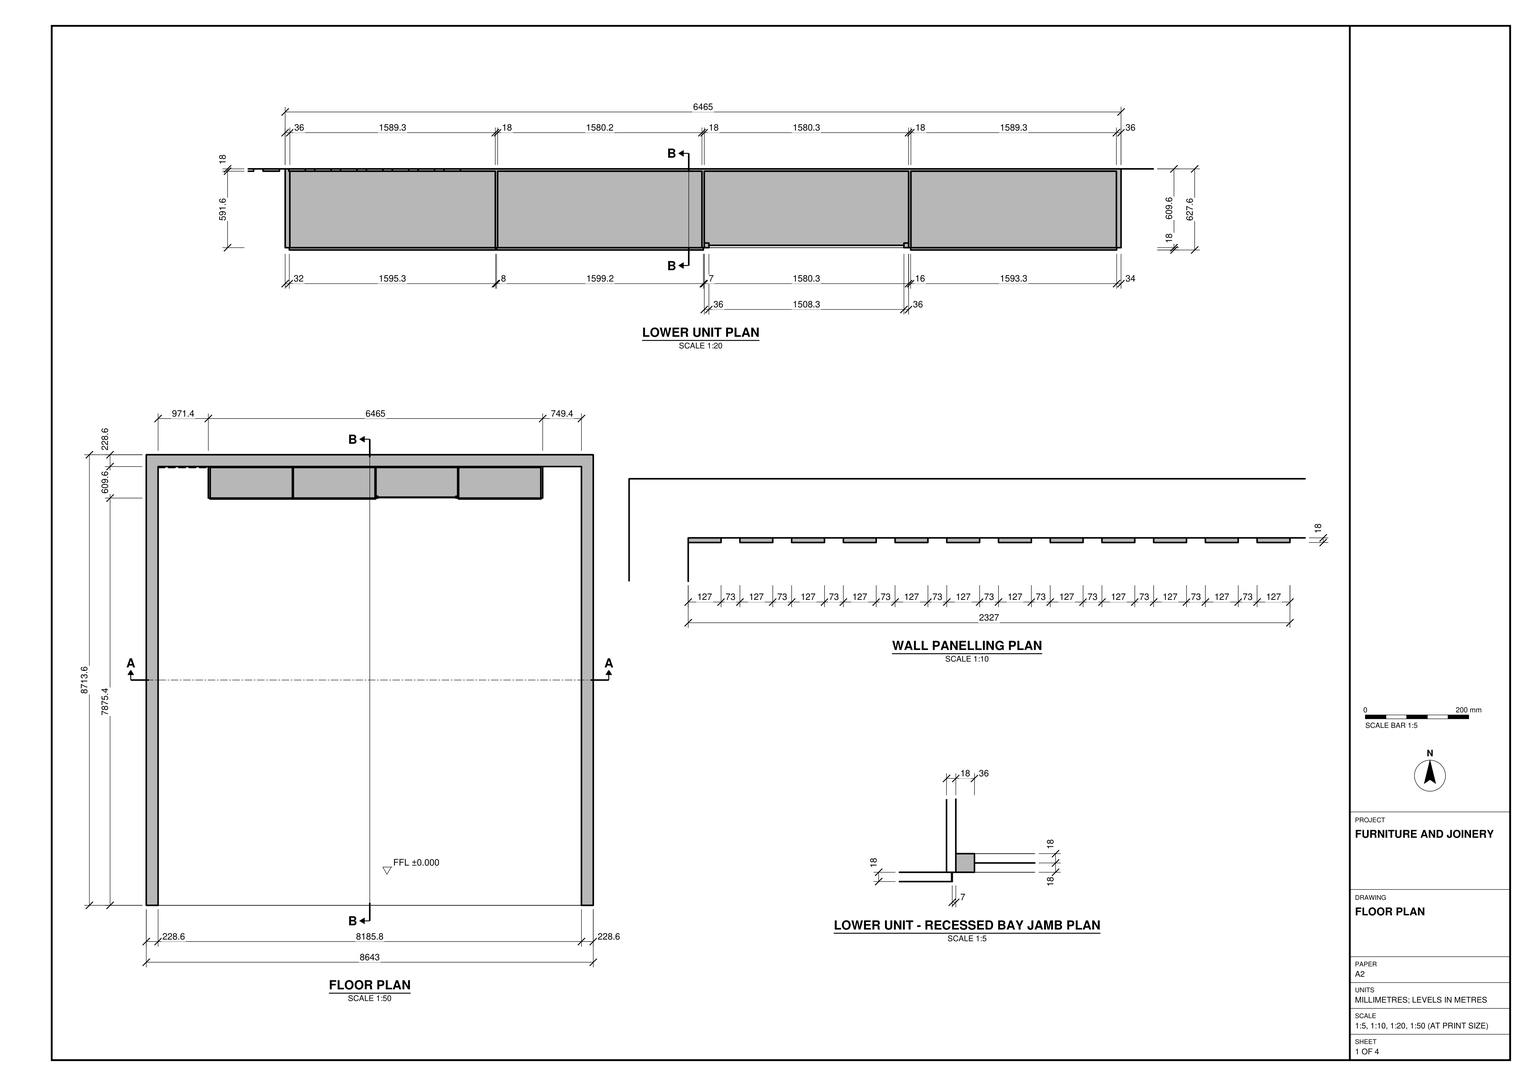
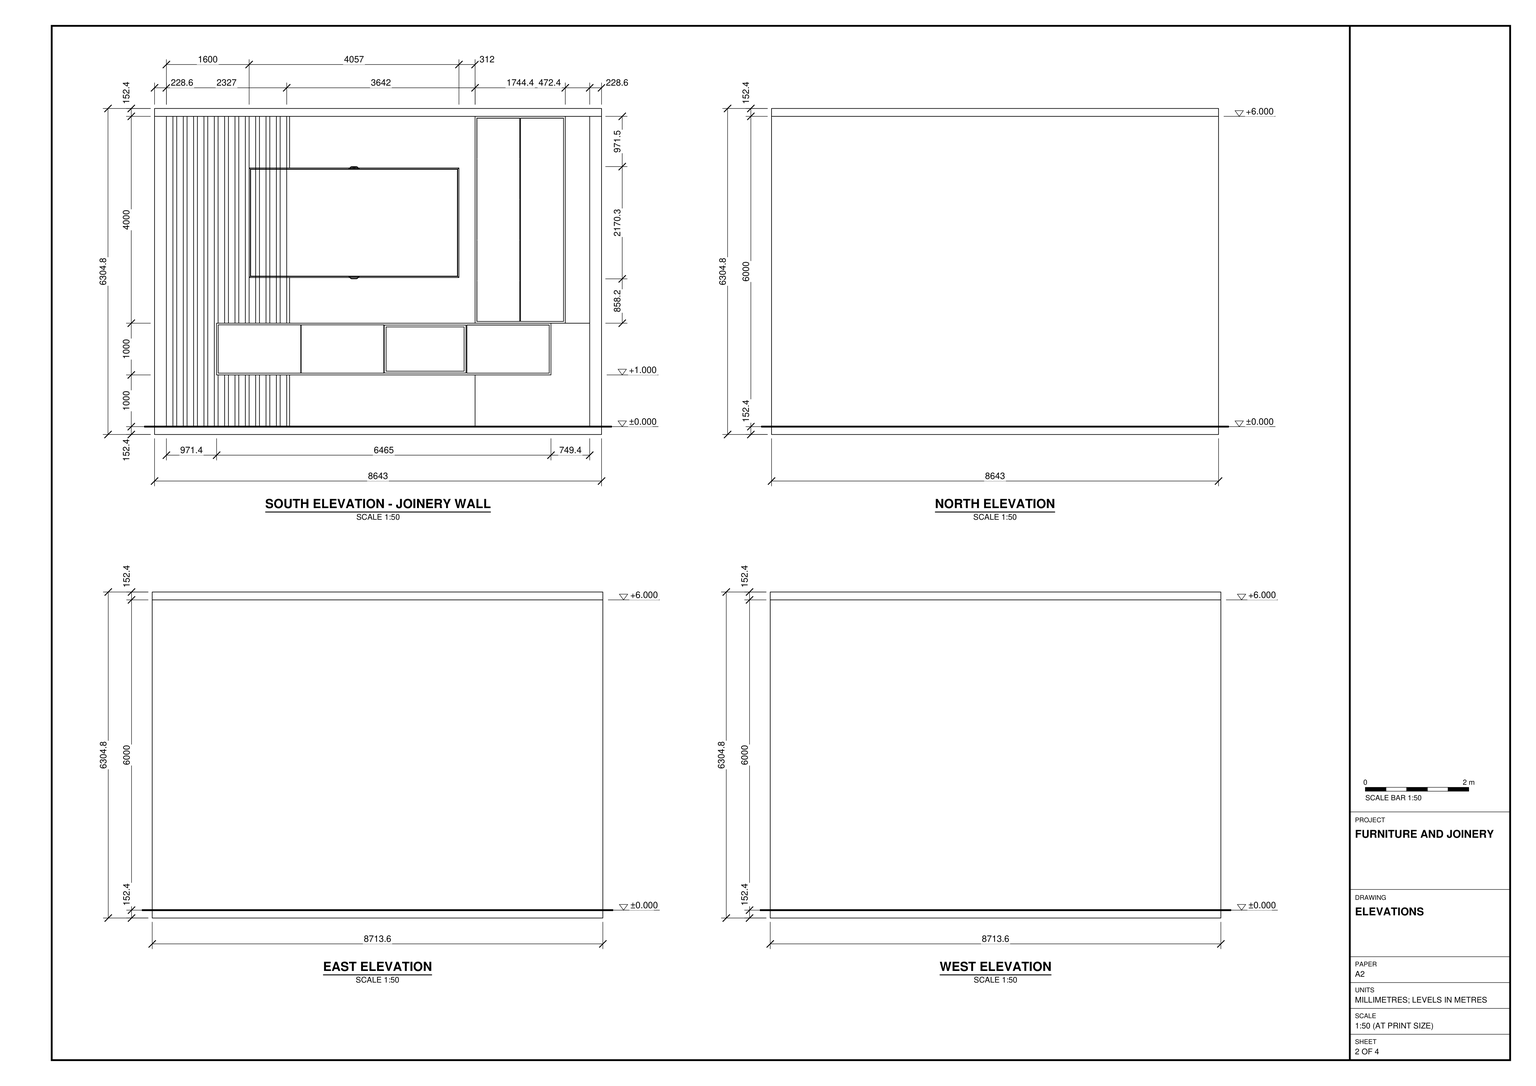
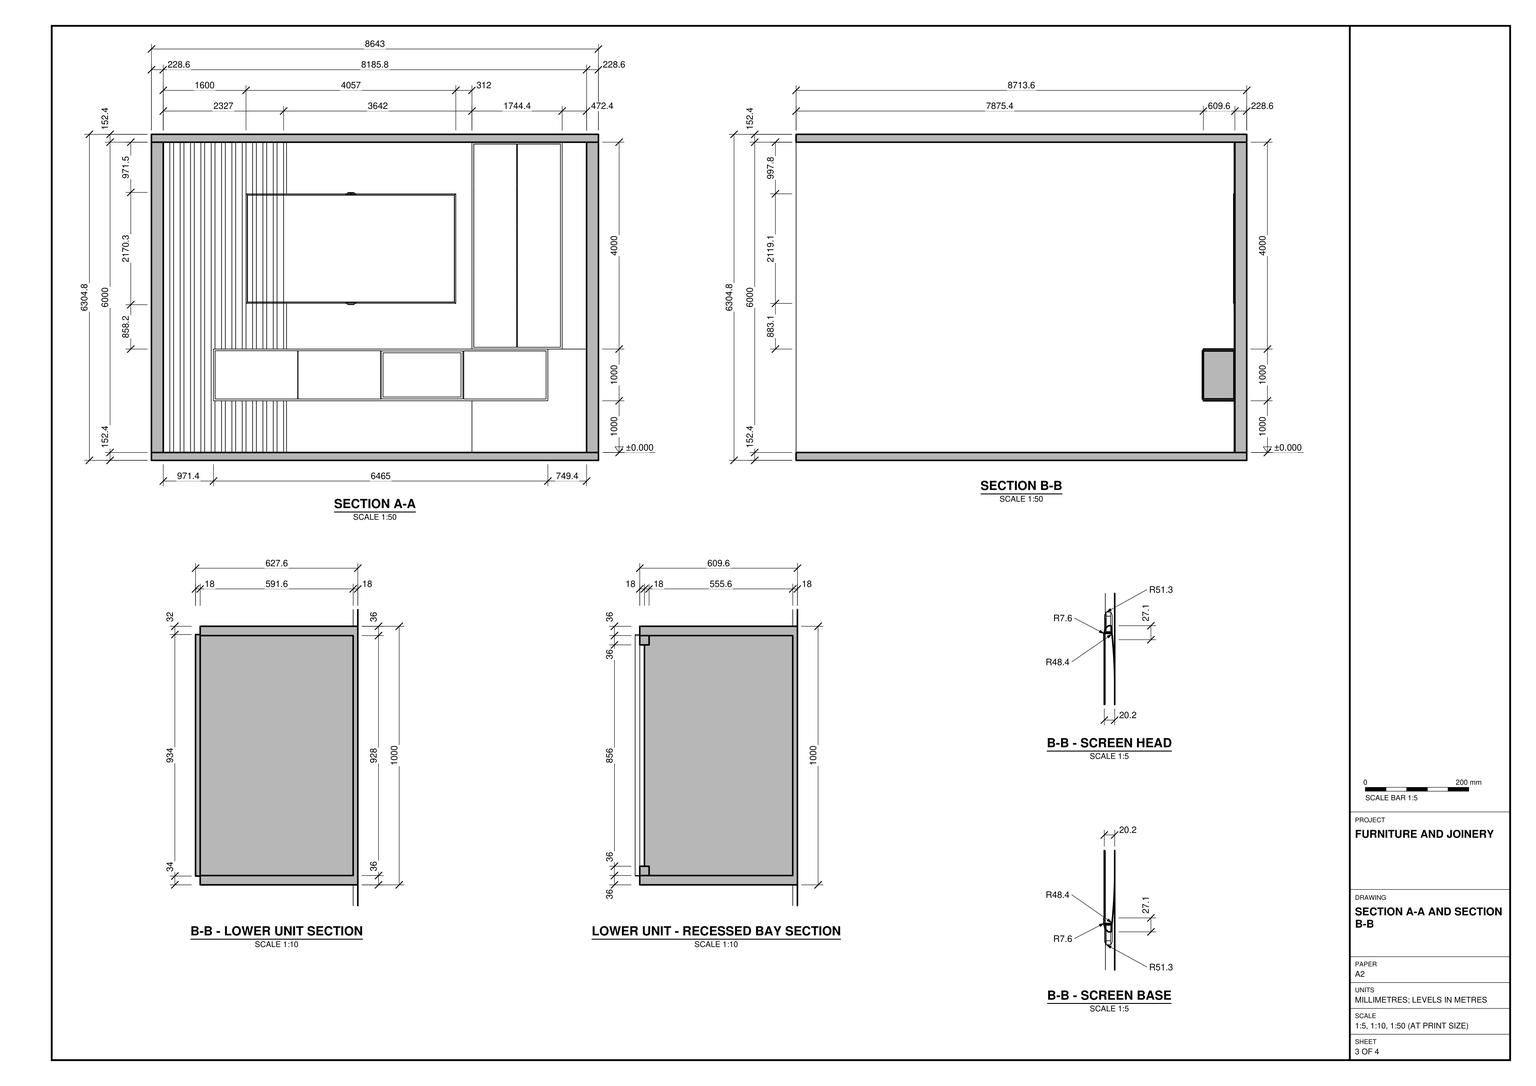
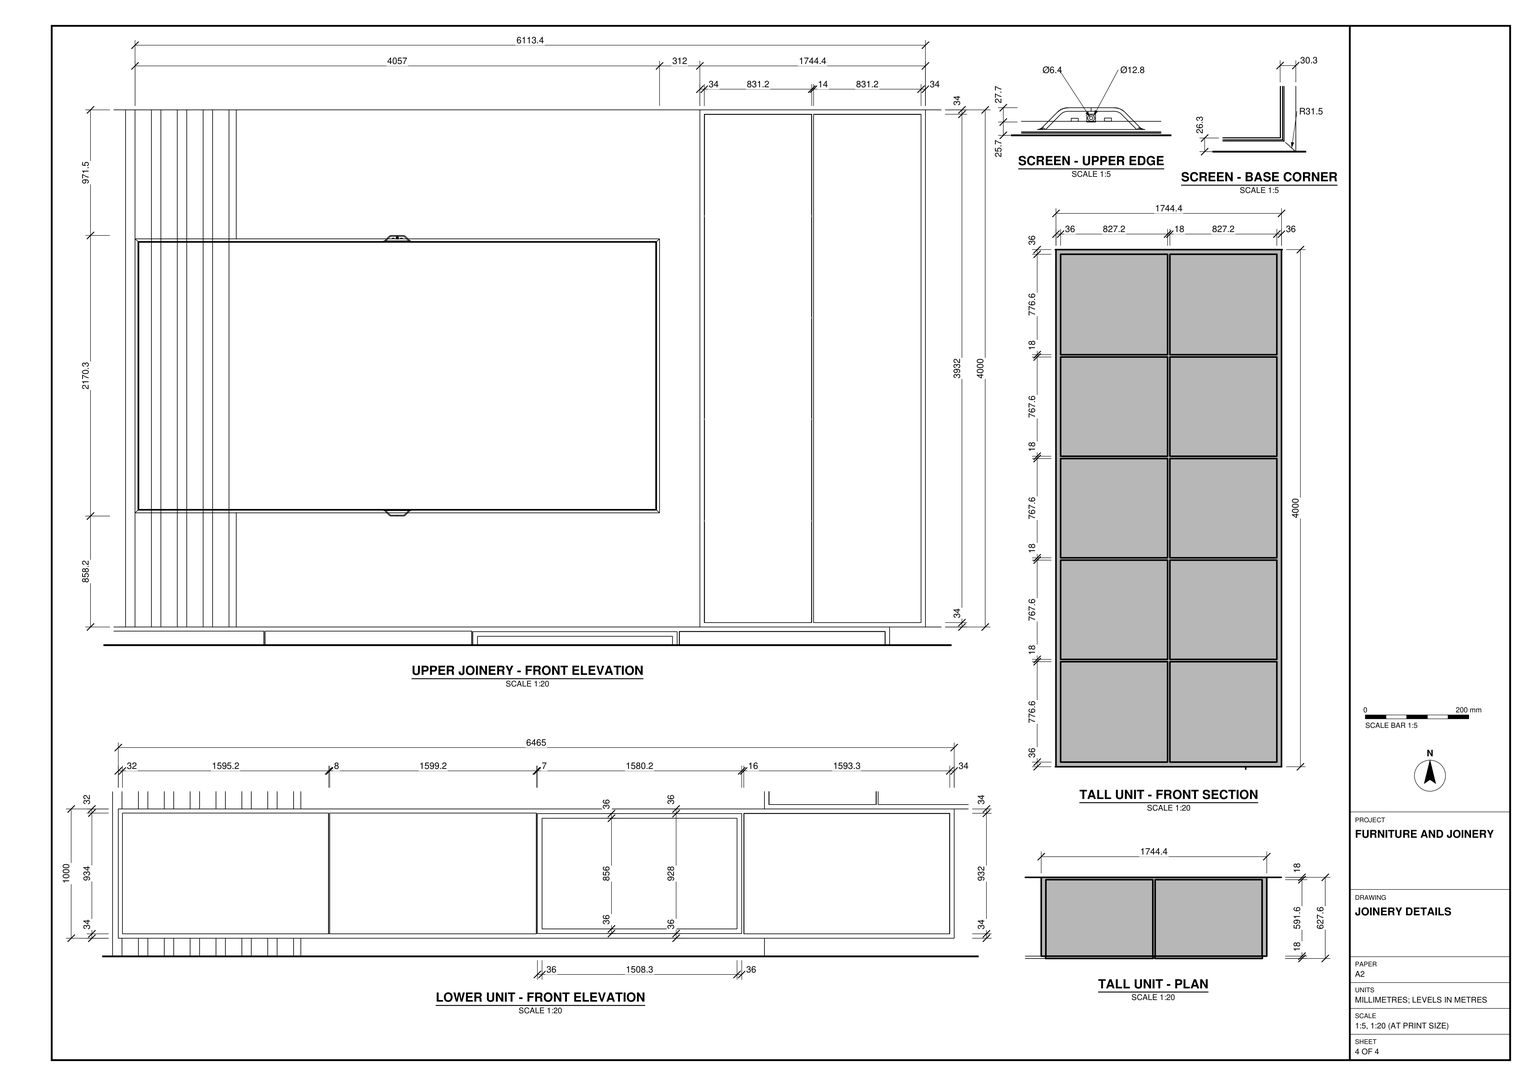
Work in millimetres in SketchUp from task_files/diagram_01.pdf. Model the open-sided room and the fitted media wall visible from its open end. The overall dimensions are 8643 mm wide, 8713.6 mm deep and 6304.8 mm high. Use the single finished floor level, ±0.000, as the 0 mm datum. Form the back and side walls at 228.6 mm thick. Include the floor slab and flat roof slab, each 152.4 mm thick, with 6000 mm clear between them.

Facing the fitted wall, start the full-height vertical panelling at the left inside corner. Follow the panelling plan for the strip widths, gaps and projection. Mount the 6465 mm lower unit across the wall with its underside 1000 mm above the floor. Divide it into four bays, with the third bay from the left recessed. Use the enlarged plan and sections to distinguish the projecting fronts from the inset face and its surrounding frame. Above the unit, place the wide screen so its left end overlaps the panelling in elevation. Model the tall divided panel to the right of the screen, extending from the top of the lower unit to the ceiling.

Keep the shell elements and each furniture or joinery piece in separate groups or components, and use components for repeated parts. Any decor or loose items shown may use suitable library components. Save one SketchUp model as output_files/open_sided_room_with_a_fitted_media_wall.skp.

# SketchUp Ruby script. Lengths in millimetres.
U = 1.mm
M = Sketchup.active_model
def pt(a) = Geom::Point3d.new(a.map { |v| v * U })
def face(e, loops, mat)
  f = e.add_face(loops[0].map { |a| pt(a) })
  loops[1..].each { |l| e.add_face(l.map { |a| pt(a) }).erase! }
  f.material = f.back_material = mat if mat
  f
end
# faces: each face lists its corners as indices into pts; further lists are holes
def faces(e, pts, list, mat = nil) = list.each { |f| face(e, (f[0].is_a?(Array) ? f : [f]).map { |l| l.map { |i| pts[i] } }, mat) }
# xy, xz, yz: faces in a plane at the given z, y or x. An outline is a flat list of corners, or four numbers for a rectangle; further outlines are holes
def ring(l) = l.size == 4 ? [[l[0], l[1]], [l[2], l[1]], [l[2], l[3]], [l[0], l[3]]] : l.each_slice(2).to_a
def flat(e, list, mat, &to3) = list.each { |f| face(e, (f[0].is_a?(Array) ? f : [f]).map { |l| ring(l).map { |u, v| to3.(u, v) } }, mat) }
def xy(e, z, list, mat = nil) = flat(e, list, mat) { |x, y| [x, y, z] }
def xz(e, y, list, mat = nil) = flat(e, list, mat) { |x, z| [x, y, z] }
def yz(e, x, list, mat = nil) = flat(e, list, mat) { |y, z| [x, y, z] }
def lines(e, pts, list) = list.each { |a, b| e.add_line(pt(pts[a]), pt(pts[b])) }
# prism: a flat outline (further loops are holes) pulled along v
def prism(e, loops, v, mat = nil)
  f = face(e, loops, mat); d = Geom::Vector3d.new(v.map { |x| x * U })
  f.pushpull(f.normal.samedirection?(d) ? d.length : -d.length)
end
def box(e, o, s, mat = nil) = prism(e, [[o, [o[0] + s[0], o[1], o[2]], [o[0] + s[0], o[1] + s[1], o[2]], [o[0], o[1] + s[1], o[2]]]], [0, 0, s[2]], mat)
def at(x, y, z, deg = 0) = Geom::Transformation.translation(pt([x, y, z])) * Geom::Transformation.rotation(ORIGIN, Z_AXIS, deg.degrees)
def axes(o, x, y, z) = Geom::Transformation.new([*x, 0, *y, 0, *z, 0, *pt(o).to_a, 1])
def part(name) = M.definitions.add(name)
# library, detail: a bought-in or finely detailed component or shape, given as its bounding box
def library(name, o, s) = part(name).tap { |d| box(d.entities, o, s) }
def detail(e, o, s) = box(e.add_group.entities, o, s)
def put(e, d, t, mat = nil) = e.add_instance(d, t).tap { |i| i.material = mat if mat }
def group(e, t, mat = nil) = e.add_group.tap { |g| g.transformation = t; g.material = mat if mat }.entities
root = M.entities
M.materials.add("[Color A02]").color = [255, 153, 153]
M.materials.add("[Color B01]").color = [255, 216, 204]
M.materials.add("[Color M04]").color = [142, 142, 142]
M.materials.add("[Color M09]").color = [0, 0, 0]
M.materials.add("[Translucent Glass Blue]").color = [100, 149, 237]
M.materials["[Translucent Glass Blue]"].alpha = 0.5
M.materials.add("[Wood Cherry Original]").color = [152, 86, 42]
c1 = library("Television screen",[0,35.9,29],[912.5,6.9,513.2])
c2 = part("Group11\#1")
box(c2.entities,[-1191.5,-3000,0],[127,6000,18])
c3 = part("Group12\#1")
box(c3.entities,[-991.5,-3000,0],[127,6000,18])
c4 = part("Group13\#1")
box(c4.entities,[-791.5,-3000,0],[127,6000,18])
c5 = part("Group14\#1")
box(c5.entities,[-591.5,-3000,0],[127,6000,18])
c6 = part("Group15\#1")
box(c6.entities,[-391.5,-3000,0],[127,6000,18])
c7 = part("Group16\#1")
xy(c7.entities,0,[[-191.5,-3000,-64.5,-2000],[-191.5,-2000,-64.5,-1000],[-191.5,-1000,-64.5,3000]])
xy(c7.entities,18,[[-191.5,-3000,-64.5,-2000],[-191.5,-2000,-64.5,-1000],[-191.5,-1000,-64.5,3000]])
xz(c7.entities,-3000,[[-191.5,0,-64.5,18]])
xz(c7.entities,3000,[[-191.5,0,-64.5,18]])
yz(c7.entities,-191.5,[[-3000,0,-2000,18],[-2000,0,-1000,18],[-1000,0,3000,18]])
yz(c7.entities,-64.5,[[-3000,0,-2000,18],[-2000,0,-1000,18],[-1000,0,3000,18]])
c8 = part("Group17\#1")
xy(c8.entities,0,[[8.5,-3000,135.5,-2000],[8.5,-2000,135.5,-1000],[8.5,-1000,135.5,3000]])
xy(c8.entities,18,[[8.5,-3000,135.5,-2000],[8.5,-2000,135.5,-1000],[8.5,-1000,135.5,3000]])
xz(c8.entities,-3000,[[8.5,0,135.5,18]])
xz(c8.entities,3000,[[8.5,0,135.5,18]])
yz(c8.entities,8.5,[[-3000,0,-2000,18],[-2000,0,-1000,18],[-1000,0,3000,18]])
yz(c8.entities,135.5,[[-3000,0,-2000,18],[-2000,0,-1000,18],[-1000,0,3000,18]])
c9 = part("Group18\#1")
xy(c9.entities,0,[[208.5,-3000,335.5,-2000],[208.5,-2000,335.5,-1000],[208.5,-1000,335.5,3000]])
xy(c9.entities,18,[[208.5,-3000,335.5,-2000],[208.5,-2000,335.5,-1000],[208.5,-1000,335.5,3000]])
xz(c9.entities,-3000,[[208.5,0,335.5,18]])
xz(c9.entities,3000,[[208.5,0,335.5,18]])
yz(c9.entities,208.5,[[-3000,0,-2000,18],[-2000,0,-1000,18],[-1000,0,3000,18]])
yz(c9.entities,335.5,[[-3000,0,-2000,18],[-2000,0,-1000,18],[-1000,0,3000,18]])
c10 = part("Group19\#1")
xy(c10.entities,0,[[408.5,-3000,535.5,-2000],[408.5,-2000,535.5,-1000],[408.5,-1000,535.5,3000]])
xy(c10.entities,18,[[408.5,-3000,535.5,-2000],[408.5,-2000,535.5,-1000],[408.5,-1000,535.5,3000]])
xz(c10.entities,-3000,[[408.5,0,535.5,18]])
xz(c10.entities,3000,[[408.5,0,535.5,18]])
yz(c10.entities,408.5,[[-3000,0,-2000,18],[-2000,0,-1000,18],[-1000,0,3000,18]])
yz(c10.entities,535.5,[[-3000,0,-2000,18],[-2000,0,-1000,18],[-1000,0,3000,18]])
c11 = part("Group20\#1")
xy(c11.entities,0,[[608.5,-3000,735.5,-2000],[608.5,-2000,735.5,-1000],[608.5,-1000,735.5,3000]])
xy(c11.entities,18,[[608.5,-3000,735.5,-2000],[608.5,-2000,735.5,-1000],[608.5,-1000,735.5,3000]])
xz(c11.entities,-3000,[[608.5,0,735.5,18]])
xz(c11.entities,3000,[[608.5,0,735.5,18]])
yz(c11.entities,608.5,[[-3000,0,-2000,18],[-2000,0,-1000,18],[-1000,0,3000,18]])
yz(c11.entities,735.5,[[-3000,0,-2000,18],[-2000,0,-1000,18],[-1000,0,3000,18]])
c12 = part("Group21\#1")
xy(c12.entities,0,[[808.5,-3000,935.5,-2000],[808.5,-2000,935.5,-1000],[808.5,-1000,935.5,3000]])
xy(c12.entities,18,[[808.5,-3000,935.5,-2000],[808.5,-2000,935.5,-1000],[808.5,-1000,935.5,3000]])
xz(c12.entities,-3000,[[808.5,0,935.5,18]])
xz(c12.entities,3000,[[808.5,0,935.5,18]])
yz(c12.entities,808.5,[[-3000,0,-2000,18],[-2000,0,-1000,18],[-1000,0,3000,18]])
yz(c12.entities,935.5,[[-3000,0,-2000,18],[-2000,0,-1000,18],[-1000,0,3000,18]])
c13 = part("Group22\#1")
xy(c13.entities,0,[[1008.5,-3000,1135.5,-2000],[1008.5,-2000,1135.5,-1000],[1008.5,-1000,1135.5,3000]])
xy(c13.entities,18,[[1008.5,-3000,1135.5,-2000],[1008.5,-2000,1135.5,-1000],[1008.5,-1000,1135.5,3000]])
xz(c13.entities,-3000,[[1008.5,0,1135.5,18]])
xz(c13.entities,3000,[[1008.5,0,1135.5,18]])
yz(c13.entities,1008.5,[[-3000,0,-2000,18],[-2000,0,-1000,18],[-1000,0,3000,18]])
yz(c13.entities,1135.5,[[-3000,0,-2000,18],[-2000,0,-1000,18],[-1000,0,3000,18]])
c14 = part("Group9\#1")
put(c14.entities,c2,at(0,0,0))
put(c14.entities,c3,at(0,0,0))
put(c14.entities,c4,at(0,0,0))
put(c14.entities,c5,at(0,0,0))
put(c14.entities,c6,at(0,0,0))
put(c14.entities,c7,at(0,0,0))
put(c14.entities,c8,at(0,0,0))
put(c14.entities,c9,at(0,0,0))
put(c14.entities,c10,at(0,0,0))
put(c14.entities,c11,at(0,0,0))
put(c14.entities,c12,at(0,0,0))
put(c14.entities,c13,at(0,0,0))
c15 = part("Group\#14")
box(c15.entities,[0,0,0],[8643,8713.6,152.4])
xz(root,7893.4,[[4477.5,-1207.6,5985.8,-351.6]],"[Translucent Glass Blue]")
put(root,c1,axes([1828.6,8356.6,455.8],[4.44606,0,0],[0,3,0],[0,0,4.2291]))
g1 = group(root,at(4441.5,7875.4,-1243.6),"[Color M04]")
xy(g1,0,[[0,0,1580.3,36]])
xy(g1,36,[[36,0,1544.3,36]])
xy(g1,892,[[36,0,1544.3,36]])
xy(g1,928,[[0,0,1580.3,36]])
xz(g1,0,[[[0,0,1580.3,928],[36,36,1544.3,892]]],"[Color M09]")
xz(g1,36,[[[0,0,1580.3,928],[36,36,1544.3,892]]])
yz(g1,0,[[0,0,36,928]])
yz(g1,36,[[0,36,36,892]])
yz(g1,1544.3,[[0,36,36,892]])
yz(g1,1580.3,[[0,0,36,928]])
g2 = group(root,at(440,8713.6,-2279.6),"[Color A02]")
xy(g2,0,[[-440,-8713.6,-440,0,8203,0,8203,-8713.6,7974.4,-8713.6,7974.4,-228.6,-211.4,-228.6,-211.4,-8713.6]])
xy(g2,6000,[[-440,-8713.6,-211.4,-8713.6,-211.4,-228.6,7974.4,-228.6,7974.4,-8713.6,8203,-8713.6,8203,0,-440,0]])
xz(g2,-8713.6,[[-440,0,-211.4,6000]])
xz(g2,-8713.6,[[7974.4,0,8203,6000]],"[Color A02]")
xz(g2,-228.6,[[2171.6,0,5757.6,1000],[5757.6,0,7974.4,0,7974.4,2000,7225,2000,7225,1000,5757.6,1000],[2171.6,2000,5757.6,6000],[5757.6,2000,7974.4,6000]])
xz(g2,-228.6,[[-211.4,0,2171.6,0,2171.6,1000,7225,1000,7225,2000,2171.6,2000,2171.6,6000,-211.4,6000]],"[Color B01]")
xz(g2,0,[[-440,0,8203,6000]])
yz(g2,-440,[[-8713.6,0,0,6000]])
yz(g2,-211.4,[[-8713.6,0,-228.6,6000]])
yz(g2,7974.4,[[-8713.6,0,-228.6,6000]],"[Color A02]")
yz(g2,8203,[[-8713.6,0,0,6000]])
g3 = group(g2,at(-211.4,-228.6,0),"[Wood Cherry Original]")
p = [[2383,0,1000],[2383,0,0],[971.4,0,1000],[971.4,0,2000],[2383,0,2000],[2383,0,6000],
  [0,0,6000],[0,0,0]]
lines(g3,p,[[0,1],[2,0],[3,2],[4,3],[5,4],[5,6],[6,7],[7,1]])
put(g3,c14,axes([1191.5,0,3000],[1,0,0],[0,0,1],[0,-1,0]))
g4 = group(g2,at(760,-228.6,1000))
xy(g4,0,[[0,-609.6,6465,0]],"[Wood Cherry Original]")
xy(g4,36,[[36,-609.6,1625.3,-18],[1643.3,-609.6,3223.5,-18],[3241.5,-609.6,4821.8,-18],[4839.8,-609.6,6429,-18]])
xy(g4,964,[[36,-609.6,1625.3,-18],[1643.3,-609.6,3223.5,-18],[3241.5,-609.6,4821.8,-18],[4839.8,-609.6,6429,-18]])
xy(g4,1000,[[0,-609.6,6465,0]],"[Wood Cherry Original]")
xz(g4,-609.6,[[[0,0,6465,1000],[36,36,36,964,1625.3,964,1625.3,36,1643.3,36,1643.3,964,3223.5,964,3223.5,36],[4839.8,36,6429,964],[3241.5,36,4821.8,964]]],"[Wood Cherry Original]")
xz(g4,-18,[[36,36,1625.3,964],[3241.5,36,4821.8,964],[4839.8,36,6429,964]])
xz(g4,-18,[[1643.3,36,3223.5,964]],"[Wood Cherry Original]")
xz(g4,0,[[0,0,6465,1000]])
yz(g4,0,[[-609.6,0,0,1000]],"[Wood Cherry Original]")
yz(g4,36,[[-609.6,36,-18,964]])
yz(g4,1625.3,[[-609.6,36,-18,964]])
yz(g4,1643.3,[[-609.6,36,-18,964]])
yz(g4,3223.5,[[-609.6,36,-18,964]])
yz(g4,3241.5,[[-609.6,36,-18,964]])
yz(g4,4821.8,[[-609.6,36,-18,964]])
yz(g4,4839.8,[[-609.6,36,-18,964]])
yz(g4,6429,[[-609.6,36,-18,964]])
yz(g4,6465,[[-609.6,0,0,1000]],"[Wood Cherry Original]")
g5 = group(g2,at(796,-838.2,1036),"[Wood Cherry Original]")
box(g5,[-4,-18,-2],[1595.3,18,934])
g6 = group(g2,at(5599.8,-838.2,1036),"[Wood Cherry Original]")
xy(g6,-2,[[-2,-18,1591.3,0]])
xy(g6,930,[[-2,-18,1591.3,0]])
xz(g6,-18,[[-2,-2,1591.3,930]])
xz(g6,0,[[-2,-2,0,0],[0,-2,1589.3,0],[1589.3,-2,1591.3,0],[-2,0,0,928],[0,0,1589.3,928],
  [1589.3,0,1589.3,928,1591.3,930,1591.3,0],[-2,928,0,930],[0,928,1589.3,930],[1589.3,928,1589.3,930,1591.3,930]])
yz(g6,-2,[[-18,-2,0,930]])
yz(g6,1591.3,[[-18,-2,0,930]])
p = [[0,-18,928],[0,0,928],[0,0,0],[0,-18,0],[1589.3,0,928],[1589.3,-18,928],
  [1589.3,-18,0],[1589.3,0,0]]
lines(g6,p,[[0,1],[2,3],[4,5],[6,7]])
g7 = group(g2,at(2403.3,-838.2,1036),"[Wood Cherry Original]")
xy(g7,-2,[[-8,-18,1591.3,0]])
xy(g7,932,[[-8,-18,1591.3,0]])
xz(g7,-18,[[-8,-2,1591.3,932]])
xz(g7,0,[[-8,-2,-4,0],[-4,-2,1589.3,0],[1589.3,-2,1591.3,0],[-8,0,-4,928],[-4,0,1589.3,928],
  [1589.3,0,1591.3,928],[-8,928,-4,932],[-4,928,1589.3,932],[1589.3,928,1591.3,932]])
yz(g7,-8,[[-18,-2,0,932]])
yz(g7,1591.3,[[-18,-2,0,928],[-18,928,0,932]])
p = [[-4,0,928],[-4,-18,928],[-4,-18,0],[-4,0,0],[1589.3,-18,928],[1589.3,0,928],
  [1589.3,-18,0],[1589.3,0,0]]
lines(g7,p,[[0,1],[2,3],[4,5],[6,7]])
g8 = group(g2,at(5757.6,-228.6,2000),"[Wood Cherry Original]")
xy(g8,0,[[0,-609.6,1467.4,0],[1467.4,-609.6,1744.4,0]])
xy(g8,36,[[36,-609.6,863.2,-18],[881.2,-609.6,1708.4,-18]])
xy(g8,812.6,[[36,-609.6,863.2,-18],[881.2,-609.6,1708.4,-18]])
xy(g8,830.6,[[36,-609.6,863.2,-18],[881.2,-609.6,1708.4,-18]])
xy(g8,1598.2,[[36,-609.6,863.2,-18],[881.2,-609.6,1708.4,-18]])
xy(g8,1616.2,[[36,-609.6,863.2,-18],[881.2,-609.6,1708.4,-18]])
xy(g8,2383.8,[[36,-609.6,863.2,-18],[881.2,-609.6,1708.4,-18]])
xy(g8,2401.8,[[36,-609.6,863.2,-18],[881.2,-609.6,1708.4,-18]])
xy(g8,3169.4,[[36,-609.6,863.2,-18],[881.2,-609.6,1708.4,-18]])
xy(g8,3187.4,[[36,-609.6,863.2,-18],[881.2,-609.6,1708.4,-18]])
xy(g8,3964,[[36,-609.6,863.2,-18],[881.2,-609.6,1708.4,-18]])
xy(g8,4000,[[0,-609.6,1744.4,0]])
xz(g8,-609.6,[[[0,0,1744.4,4000],[36,1616.2,36,3169.4,863.2,3169.4,863.2,2401.8,36,2401.8,36,2383.8,863.2,2383.8,863.2,1616.2],[881.2,1616.2,881.2,2383.8,1708.4,2383.8,1708.4,2401.8,881.2,2401.8,881.2,3169.4,1708.4,3169.4,1708.4,1616.2],[36,36,863.2,812.6],[36,3187.4,863.2,3964],[881.2,36,1708.4,812.6],[881.2,3187.4,1708.4,3964],[36,830.6,863.2,1598.2],[881.2,830.6,1708.4,1598.2]]])
xz(g8,-18,[[36,36,863.2,812.6],[881.2,36,1708.4,812.6],[36,830.6,863.2,1598.2],[881.2,830.6,1708.4,1598.2],[36,1616.2,863.2,2383.8],
  [881.2,1616.2,1708.4,2383.8],[36,2401.8,863.2,3169.4],[881.2,2401.8,1708.4,3169.4],[36,3187.4,863.2,3964],[881.2,3187.4,1708.4,3964]])
xz(g8,0,[[0,0,1744.4,4000]])
yz(g8,0,[[-609.6,0,0,4000]])
yz(g8,36,[[-609.6,36,-18,812.6],[-609.6,830.6,-18,1598.2],[-609.6,1616.2,-18,2383.8],[-609.6,2401.8,-18,3169.4],[-609.6,3187.4,-18,3964]])
yz(g8,863.2,[[-609.6,36,-18,812.6],[-609.6,830.6,-18,1598.2],[-609.6,1616.2,-18,2383.8],[-609.6,2401.8,-18,3169.4],[-609.6,3187.4,-18,3964]])
yz(g8,881.2,[[-609.6,36,-18,812.6],[-609.6,830.6,-18,1598.2],[-609.6,1616.2,-18,2383.8],[-609.6,2401.8,-18,3169.4],[-609.6,3187.4,-18,3964]])
yz(g8,1708.4,[[-609.6,36,-18,812.6],[-609.6,830.6,-18,1598.2],[-609.6,1616.2,-18,2383.8],[-609.6,2401.8,-18,3169.4],[-609.6,3187.4,-18,3964]])
yz(g8,1744.4,[[-609.6,0,0,4000]])
g9 = group(g2,at(5793.6,-838.2,2036),"[Translucent Glass Blue]")
box(g9,[-2,-18,-2],[831.2,18,3932])
g10 = group(g2,at(6638.8,-838.2,2036),"[Translucent Glass Blue]")
box(g10,[-2,-18,-2],[831.2,18,3932])
put(root,c15,at(0,0,3720.4))
put(root,c15,at(0,0,-2432))
